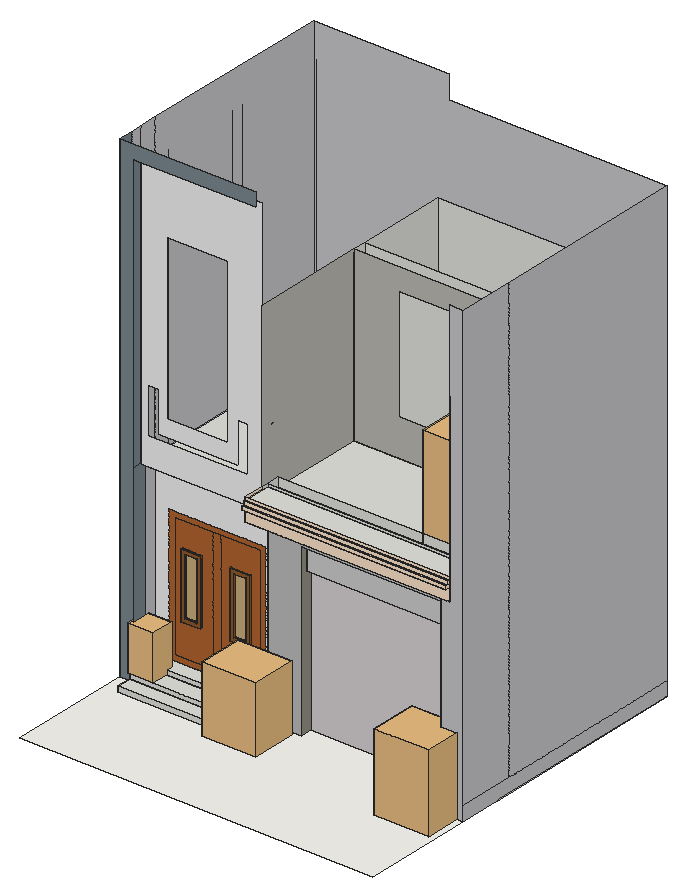
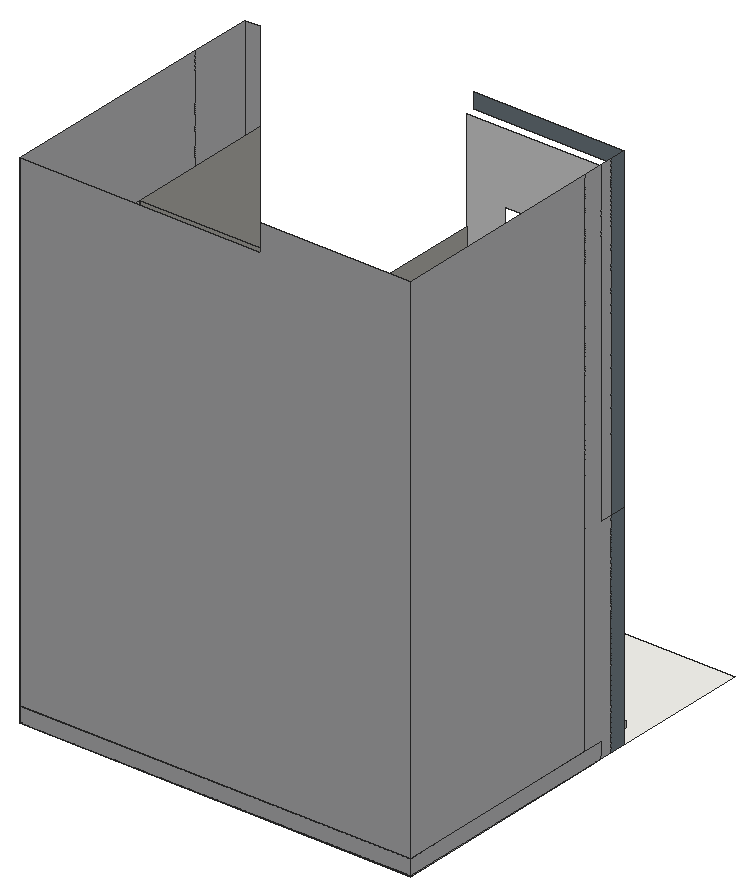
# SketchUp Ruby script. Lengths in inches.
U = 1.inch
M = Sketchup.active_model
def pt(a) = Geom::Point3d.new(a.map { |v| v * U })
def face(e, loops, mat)
  f = e.add_face(loops[0].map { |a| pt(a) })
  loops[1..].each { |l| e.add_face(l.map { |a| pt(a) }).erase! }
  f.material = f.back_material = mat if mat
  f
end
# faces: each face lists its corners as indices into pts; further lists are holes
def faces(e, pts, list, mat = nil) = list.each { |f| face(e, (f[0].is_a?(Array) ? f : [f]).map { |l| l.map { |i| pts[i] } }, mat) }
# xy, xz, yz: faces in a plane at the given z, y or x. An outline is a flat list of corners, or four numbers for a rectangle; further outlines are holes
def ring(l) = l.size == 4 ? [[l[0], l[1]], [l[2], l[1]], [l[2], l[3]], [l[0], l[3]]] : l.each_slice(2).to_a
def flat(e, list, mat, &to3) = list.each { |f| face(e, (f[0].is_a?(Array) ? f : [f]).map { |l| ring(l).map { |u, v| to3.(u, v) } }, mat) }
def xy(e, z, list, mat = nil) = flat(e, list, mat) { |x, y| [x, y, z] }
def xz(e, y, list, mat = nil) = flat(e, list, mat) { |x, z| [x, y, z] }
def yz(e, x, list, mat = nil) = flat(e, list, mat) { |y, z| [x, y, z] }
def lines(e, pts, list) = list.each { |a, b| e.add_line(pt(pts[a]), pt(pts[b])) }
# prism: a flat outline (further loops are holes) pulled along v
def prism(e, loops, v, mat = nil)
  f = face(e, loops, mat); d = Geom::Vector3d.new(v.map { |x| x * U })
  f.pushpull(f.normal.samedirection?(d) ? d.length : -d.length)
end
def box(e, o, s, mat = nil) = prism(e, [[o, [o[0] + s[0], o[1], o[2]], [o[0] + s[0], o[1] + s[1], o[2]], [o[0], o[1] + s[1], o[2]]]], [0, 0, s[2]], mat)
def at(x, y, z, deg = 0) = Geom::Transformation.translation(pt([x, y, z])) * Geom::Transformation.rotation(ORIGIN, Z_AXIS, deg.degrees)
def axes(o, x, y, z) = Geom::Transformation.new([*x, 0, *y, 0, *z, 0, *pt(o).to_a, 1])
def part(name) = M.definitions.add(name)
# library, detail: a bought-in or finely detailed component or shape, given as its bounding box
def library(name, o, s) = part(name).tap { |d| box(d.entities, o, s) }
def detail(e, o, s) = box(e.add_group.entities, o, s)
def put(e, d, t, mat = nil) = e.add_instance(d, t).tap { |i| i.material = mat if mat }
def group(e, t, mat = nil) = e.add_group.tap { |g| g.transformation = t; g.material = mat if mat }.entities
root = M.entities
M.materials.add("[Blinds Cellular White]2").color = [217, 211, 213]
M.materials.add("[Blinds Vertical Pattern]").color = [189, 189, 191]
M.materials.add("[Carrera Marble]").color = [207, 207, 207]
M.materials.add("[Cladding Siding White]").color = [242, 242, 242]
M.materials.add("[Color C01]").color = [255, 229, 204]
M.materials.add("[Formica Graystone]").color = [149, 146, 135]
M.materials.add("[Formica Laminate Light]").color = [213, 189, 164]
M.materials.add("[Formica Speckled Grey]").color = [123, 137, 145]
M.materials.add("[Pavers Driveway Brick]").color = [249, 248, 243]
M.materials.add("[Polished Concrete New]").color = [200, 200, 203]
M.materials.add("[Terrazzo Tile Light]").color = [188, 186, 180]
M.materials.add("[Wood Cherry Original]").color = [178, 100, 49]
M.materials.add("[Wood Floor Light]").color = [204, 176, 127]
M.materials.add("[Wood Floor Parquet]").color = [145, 89, 39]
c1 = library("chau cay",[-24.34,-109.24,0],[56.46,62.58,79.69])
c2 = library("Sem+nome",[-20.92,-6.25,0],[92.79,42.83,52.11])
c3 = library("Flora+17",[-57.52,158.6,-38.64],[66.99,62.88,77.28])
xy(root,0,[[0,856.59,1944.31,2018.8]])
xy(root,2.5,[[77.12,577.64,746.18,657.3],[1822.57,617.28,1944.31,688.65],[77.12,657.3,746.18,688.65],[0,688.65,77.12,834.03],[1822.57,688.65,1822.57,834.03,0,834.03,0,856.59,1944.31,856.59,1944.31,688.65],
  [77.12,688.65,746.18,749.64],[77.12,749.64,746.18,834.03],[746.18,769.97,935.56,834.03],[1728.74,769.97,1822.57,834.03],[0,856.59,1944.31,2018.8]])
xy(root,2.5,[[0,0,0,688.65,77.12,688.65,77.12,577.64,746.18,577.64,746.18,769.97,935.56,769.97,935.56,834.03,1728.74,834.03,1728.74,769.97,1822.57,769.97,1822.57,617.28,1944.31,617.28,1944.31,0]],"[Pavers Driveway Brick]")
xy(root,32,[[77.12,577.64,746.18,657.3]])
xy(root,56.75,[[77.12,657.3,746.18,749.64]])
xy(root,80.25,[[0,930.73,0,2018.8,1944.31,2018.8,1944.31,930.73,1870.17,930.73,1870.17,1944.66,74.14,1944.66,74.14,930.73],[74.14,930.73,1870.17,1367.21],[74.14,1367.21,1870.17,1437.7],[74.14,1437.7,1870.17,1944.66]])
xy(root,81.6875,[[77.12,749.64,746.18,834.03]])
xy(root,294.7,[[227.2,834.03,334.7,837.4]])
xy(root,294.7,[[227.2,824.72,334.7,834.03],[495.57,824.72,603.07,834.03]],"[Wood Floor Parquet]")
xy(root,313.68,[[246.18,834.03,315.72,837.4]])
xy(root,313.68,[[246.18,824.72,315.72,834.03],[514.55,824.72,584.09,834.03]],"[Wood Floor Parquet]")
xy(root,632.29,[[246.18,834.03,315.72,837.4]])
xy(root,632.29,[[246.18,824.72,315.72,834.03],[514.55,824.72,584.09,834.03]],"[Wood Floor Parquet]")
xy(root,651.27,[[227.2,834.03,334.7,837.4]])
xy(root,651.27,[[227.2,824.72,334.7,834.03],[495.57,824.72,603.07,834.03]],"[Wood Floor Parquet]")
xy(root,800.43,[[935.56,802.78,1728.74,834.03]],"[Carrera Marble]")
xy(root,935.1875,[[935.56,802.78,1728.74,834.03]],"[Carrera Marble]")
xy(root,935.1875,[[935.56,769.97,1728.74,802.78]],"[Formica Graystone]")
xy(root,1060.1875,[[1822.57,617.28,1870.17,617.28,1870.17,930.73,74.14,930.73,74.14,769.97,77.12,769.97,77.12,834.03,1822.57,834.03],[971.14,654.98,962.89,656.07,955.2,659.25,948.6,664.32,943.53,670.92,940.35,678.61,939.26,686.86,940.35,695.1,943.53,702.79,948.6,709.39,955.2,714.46,962.89,717.64,971.14,718.73,979.39,717.64,987.07,714.46,993.68,709.39,998.74,702.79,1001.93,695.1,1003.01,686.86,1001.93,678.61,998.74,670.92,993.68,664.32,987.07,659.25,979.39,656.07],[1617.57,654.98,1609.32,656.07,1601.64,659.25,1595.03,664.32,1589.97,670.92,1586.78,678.61,1585.7,686.86,1586.78,695.1,1589.97,702.79,1595.03,709.39,1601.64,714.46,1609.32,717.64,1617.57,718.73,1625.82,717.64,1633.51,714.46,1640.11,709.39,1645.18,702.79,1648.36,695.1,1649.45,686.86,1648.36,678.61,1645.18,670.92,1640.11,664.32,1633.51,659.25,1625.82,656.07],[77.12,733.78,746.18,834.03],[746.18,769.97,1822.57,834.03],
  [74.14,930.73,1870.17,1367.21],[74.14,1367.21,1870.17,1437.7],[74.14,1437.7,1870.17,1944.66]])
xy(root,1060.1875,[[[746.18,617.28,1822.57,769.97],[971.14,654.98,979.39,656.07,987.07,659.25,993.68,664.32,998.74,670.92,1001.93,678.61,1003.01,686.86,1001.93,695.1,998.74,702.79,993.68,709.39,987.07,714.46,979.39,717.64,971.14,718.73,962.89,717.64,955.2,714.46,948.6,709.39,943.53,702.79,940.35,695.1,939.26,686.86,940.35,678.61,943.53,670.92,948.6,664.32,955.2,659.25,962.89,656.07],[1617.57,654.98,1625.82,656.07,1633.51,659.25,1640.11,664.32,1645.18,670.92,1648.36,678.61,1649.45,686.86,1648.36,695.1,1645.18,702.79,1640.11,709.39,1633.51,714.46,1625.82,717.64,1617.57,718.73,1609.32,717.64,1601.64,714.46,1595.03,709.39,1589.97,702.79,1586.78,695.1,1585.7,686.86,1586.78,678.61,1589.97,670.92,1595.03,664.32,1601.64,659.25,1609.32,656.07]]],"[Formica Laminate Light]")
xy(root,1130.875,[[746.18,844.59,1870.17,1367.21],[746.18,1367.21,1870.17,1437.7],[746.18,1437.7,1870.17,1944.66]])
xy(root,1131.125,[[746.18,592.22,1870.17,617.28],[746.18,617.28,1870.17,769.97]])
xy(root,1148.625,[[746.18,603.97,1870.17,769.97]])
xy(root,1148.625,[[746.18,592.22,1870.17,603.97]],"[Color C01]")
xy(root,1166.1875,[[746.18,617.28,1870.17,769.97]])
xy(root,1166.1875,[[746.18,603.97,1870.17,617.28]],"[Color C01]")
xz(root,577.64,[[77.12,2.5,746.18,32]])
xz(root,592.22,[[746.18,1131.125,1870.17,1148.625]],"[Color C01]")
xz(root,603.97,[[746.18,1148.625,1870.17,1166.1875]],"[Color C01]")
xz(root,617.28,[[746.18,1060.1875,1870.17,1131.125],[746.18,1166.1875,1870.17,1179.9375]],"[Color C01]")
xz(root,617.28,[[1822.57,2.5,1944.31,2.5,1944.31,2522.1875,1870.17,2522.1875,1870.17,1060.1875,1822.57,1060.1875]],"[Polished Concrete New]")
xz(root,657.3,[[77.12,2.5,746.18,32],[77.12,32,746.18,56.75]])
xz(root,688.65,[[0,2.5,77.12,2.5,77.12,2578.28,746.18,2578.28,746.18,2654.3125,0,2654.3125]],"[Formica Speckled Grey]")
xz(root,733.78,[[[77.12,1060.1875,746.18,2578.28],[218.87,1330.35,559.3,2229.35],[114.55,1210.6875,114.55,1463.4375,176.52,1463.4375,176.52,1243.125,613.71,1243.125,613.71,1463.4375,668.12,1463.4375,668.12,1210.6875]]],"[Cladding Siding White]")
xz(root,749.64,[[77.12,2.5,746.18,56.75],[77.12,56.75,746.18,81.6875]])
xz(root,769.97,[[746.18,1131.125,1870.17,1148.625],[746.18,1148.625,1870.17,1166.1875],[746.18,1166.1875,1870.17,1179.9375]])
xz(root,769.97,[[746.18,2.5,935.56,2.5,935.56,935.1875,1728.74,935.1875,1728.74,2.5,1822.57,2.5,1822.57,1060.1875,746.18,1060.1875]],"[Blinds Vertical Pattern]")
xz(root,802.78,[[935.56,800.43,1728.74,935.1875]],"[Carrera Marble]")
xz(root,824.72,[[[227.2,294.7,334.7,651.27],[246.18,313.68,315.72,632.29]],[[495.57,294.7,603.07,651.27],[514.55,313.68,584.09,632.29]]],"[Wood Floor Parquet]")
xz(root,834.03,[[77.12,2.5,746.18,80.25],[746.18,2.5,746.18,1060.1875,1822.57,1060.1875,1822.57,2.5,1728.74,2.5,1728.74,935.1875,935.56,935.1875,935.56,2.5],[77.12,80.25,154.02,81.6875],[154.02,80.25,687.02,81.6875],[687.02,80.25,746.18,81.6875],
  [[227.2,294.7,334.7,651.27],[246.18,313.68,315.72,632.29]],[[495.57,294.7,603.07,651.27],[514.55,313.68,584.09,632.29]]])
xz(root,834.03,[[935.56,2.5,1728.74,800.43]],"[Blinds Cellular White]2")
xz(root,834.03,[[77.12,81.6875,154.02,81.6875,154.02,821.9375,687.02,821.9375,687.02,81.6875,746.18,81.6875,746.18,1060.1875,77.12,1060.1875]],"[Cladding Siding White]")
xz(root,834.03,[[[154.02,81.6875,687.02,821.9375],[183.68,109.91,657.36,792.28]],[[183.68,109.91,395.5625,792.28],[227.2,294.7,334.7,651.27]],[395.5625,109.91,440.89,792.28],[[440.89,109.91,657.36,792.28],[495.57,294.7,603.07,651.27]]],"[Wood Cherry Original]")
xz(root,834.03,[[246.18,313.68,315.72,632.29],[514.55,313.68,584.09,632.29]],"[Wood Floor Light]")
xz(root,837.4,[[[227.2,294.7,334.7,651.27],[246.18,313.68,315.72,632.29]]])
xz(root,844.59,[[746.18,1130.875,1870.17,1179.9375]])
xz(root,856.59,[[0,0,1944.31,2.5]])
xz(root,930.73,[[74.14,80.25,1870.17,1060.1875]])
xz(root,1367.21,[[74.14,80.25,1870.17,1060.1875]])
xz(root,1367.21,[[[746.18,1130.875,1870.17,2073.3125],[988.74,1330.6,1613.49,1955.35]]],"[Terrazzo Tile Light]")
xz(root,1437.7,[[74.14,80.25,1870.17,1060.1875],[746.18,1130.875,1870.17,2073.3125]])
xz(root,1944.66,[[74.14,80.25,1870.17,1060.1875],[746.18,1130.875,1870.17,2073.3125]])
xz(root,2018.8,[[0,0,1944.31,2.5]])
xz(root,2018.8,[[0,2.5,1944.31,80.25],[0,80.25,0,2654.3125,746.18,2654.3125,746.18,2522.1875,1944.31,2522.1875,1944.31,80.25]],"[Polished Concrete New]")
yz(root,0,[[856.59,0,2018.8,2.5]])
yz(root,0,[[688.65,2.5,769.97,1060.1875],[688.65,1060.1875,769.97,2654.3125]],"[Formica Speckled Grey]")
yz(root,0,[[769.97,2.5,769.97,1060.1875,834.03,1060.1875,834.03,2654.3125,930.73,2654.3125,930.73,80.25,834.03,80.25,834.03,2.5],[834.03,2.5,2018.8,80.25],[930.73,80.25,2018.8,2654.3125],[769.97,1060.1875,834.03,2654.3125]],"[Polished Concrete New]")
yz(root,74.14,[[930.73,80.25,1367.21,1060.1875],[1367.21,80.25,1437.7,1060.1875],[1437.7,80.25,1944.66,1060.1875]])
yz(root,77.12,[[577.64,2.5,657.3,32],[657.3,2.5,688.65,56.75],[688.65,2.5,749.64,56.75],[749.64,2.5,769.97,81.6875],[769.97,2.5,834.03,81.6875],
  [733.78,1060.1875,769.97,2578.28]])
yz(root,77.12,[[688.65,56.75,749.64,56.75,749.64,81.6875,769.97,81.6875,769.97,1060.1875,688.65,1060.1875],[688.65,1060.1875,733.78,2578.28]],"[Formica Speckled Grey]")
yz(root,77.12,[[769.97,81.6875,834.03,1060.1875]],"[Polished Concrete New]")
yz(root,227.2,[[834.03,294.7,837.4,651.27]])
yz(root,227.2,[[824.72,294.7,834.03,651.27]],"[Wood Floor Parquet]")
yz(root,246.18,[[834.03,313.68,837.4,632.29]])
yz(root,246.18,[[824.72,313.68,834.03,632.29]],"[Wood Floor Parquet]")
yz(root,315.72,[[834.03,313.68,837.4,632.29]])
yz(root,315.72,[[824.72,313.68,834.03,632.29]],"[Wood Floor Parquet]")
yz(root,334.7,[[834.03,294.7,837.4,651.27]])
yz(root,334.7,[[824.72,294.7,834.03,651.27]],"[Wood Floor Parquet]")
yz(root,495.57,[[824.72,294.7,834.03,651.27]],"[Wood Floor Parquet]")
yz(root,514.55,[[824.72,313.68,834.03,632.29]],"[Wood Floor Parquet]")
yz(root,584.09,[[824.72,313.68,834.03,632.29]],"[Wood Floor Parquet]")
yz(root,603.07,[[824.72,294.7,834.03,651.27]],"[Wood Floor Parquet]")
yz(root,746.18,[[577.64,2.5,657.3,32],[657.3,2.5,749.64,56.75],[749.64,2.5,769.97,81.6875],[769.97,2.5,834.03,80.25],[769.97,80.25,834.03,81.6875],
  [733.78,1130.875,844.59,1130.875,844.59,1179.9375,769.97,1179.9375,769.97,1131.125,733.78,1131.125],[1367.21,1130.875,1437.7,2073.3125],[1437.7,1130.875,1944.66,2073.3125],[733.78,1131.125,769.97,1148.625],[733.78,1148.625,769.97,1166.1875],
  [733.78,1166.1875,769.97,1179.9375]])
yz(root,746.18,[[617.28,1060.1875,733.78,1131.125],[592.22,1131.125,733.78,1148.625],[603.97,1148.625,733.78,1166.1875],[617.28,1166.1875,733.78,1179.9375]],"[Color C01]")
yz(root,746.18,[[769.97,81.6875,834.03,1060.1875]],"[Polished Concrete New]")
yz(root,746.18,[[[844.59,1130.875,1367.21,1130.875,1367.21,2073.3125,733.78,2073.3125,733.78,1179.9375,844.59,1179.9375],[803.39,1455.01,801.4,1455.27,799.55,1456.04,797.96,1457.26,796.73,1458.85,795.97,1460.71,795.71,1462.7,795.97,1464.6875,796.73,1466.54,797.96,1468.13,799.55,1469.35,801.4,1470.12,803.39,1470.38,805.38,1470.12,807.24,1469.35,808.83,1468.13,810.05,1466.54,810.82,1464.6875,811.08,1462.7,810.82,1460.71,810.05,1458.85,808.83,1457.26,807.24,1456.04,805.38,1455.27]]],"[Terrazzo Tile Light]")
yz(root,935.56,[[802.78,800.43,834.03,935.1875]],"[Carrera Marble]")
yz(root,935.56,[[769.97,2.5,834.03,2.5,834.03,800.43,802.78,800.43,802.78,935.1875,769.97,935.1875]],"[Formica Graystone]")
yz(root,1728.74,[[802.78,800.43,834.03,935.1875]],"[Carrera Marble]")
yz(root,1728.74,[[769.97,2.5,769.97,935.1875,802.78,935.1875,802.78,800.43,834.03,800.43,834.03,2.5]],"[Formica Graystone]")
yz(root,1822.57,[[769.97,2.5,834.03,1060.1875]])
yz(root,1822.57,[[617.28,2.5,769.97,1060.1875]],"[Polished Concrete New]")
yz(root,1870.17,[[930.73,80.25,1367.21,1060.1875],[1367.21,80.25,1437.7,1060.1875],[1437.7,80.25,1944.66,1060.1875],[617.28,1060.1875,930.73,1060.1875,930.73,1130.875,844.59,1130.875,844.59,1179.9375,769.97,1179.9375,769.97,1131.125,617.28,1131.125],[930.73,1060.1875,1367.21,1130.875],
  [1367.21,1060.1875,1437.7,1130.875],[1437.7,1060.1875,1944.66,1130.875],[1367.21,1130.875,1437.7,2073.3125],[1437.7,1130.875,1944.66,2073.3125],[617.28,1131.125,769.97,1148.625],
  [617.28,1148.625,769.97,1166.1875],[617.28,1166.1875,769.97,1179.9375]])
yz(root,1870.17,[[592.22,1131.125,617.28,1148.625],[603.97,1148.625,617.28,1166.1875]],"[Color C01]")
yz(root,1870.17,[[[844.59,1130.875,844.59,1179.9375,617.28,1179.9375,617.28,2073.3125,1367.21,2073.3125,1367.21,1130.875],[803.39,1455.01,805.38,1455.27,807.24,1456.04,808.83,1457.26,810.05,1458.85,810.82,1460.71,811.08,1462.7,810.82,1464.6875,810.05,1466.54,808.83,1468.13,807.24,1469.35,805.38,1470.12,803.39,1470.38,801.4,1470.12,799.55,1469.35,797.96,1468.13,796.73,1466.54,795.97,1464.6875,795.71,1462.7,795.97,1460.71,796.73,1458.85,797.96,1457.26,799.55,1456.04,801.4,1455.27]]],"[Terrazzo Tile Light]")
yz(root,1944.31,[[856.59,0,2018.8,2.5]])
yz(root,1944.31,[[617.28,2.5,2018.8,80.25],[617.28,80.25,930.73,2522.1875],[930.73,80.25,2018.8,2522.1875]],"[Polished Concrete New]")
p = [[74.14,834.03,1060.1875],[74.14,834.03,2522.1875],[74.14,930.73,1060.1875],[74.14,930.73,2522.1875],[74.14,1367.21,1060.1875],[74.14,1367.21,2522.1875],
  [74.14,1437.7,1060.1875],[74.14,1437.7,2522.1875],[74.14,1944.66,1060.1875],[74.14,1944.66,2522.1875]]
lines(root,p,[[0,1],[2,3],[4,5],[6,7],[8,9]])
put(root,c1,axes([1740.99,875.45,2.5],[5.3618,0,0],[0,4.1292,0],[0,0,5.3352]))
put(root,c2,axes([667.04,537.7,2.5],[3.20983,0,0],[0,5.79193,0],[0,0,7]))
put(root,c3,axes([187.05,340.1,179.63],[2.07633,0,0],[0,2,0],[0,0,3.18]))
put(root,c1,axes([1674.08,1295.67,1130.875],[5.3618,0,0],[0,4.1292,0],[0,0,7.02]))
